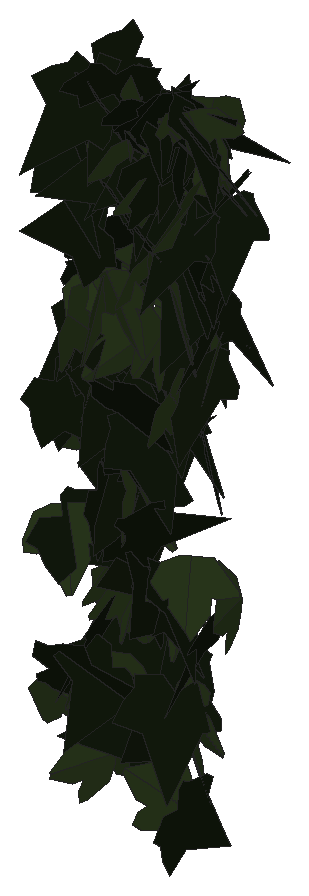
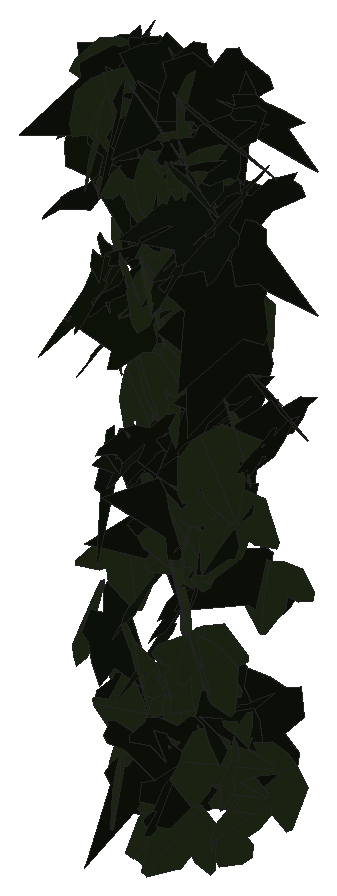
# SketchUp Ruby script. Lengths in inches.
U = 1.inch
M = Sketchup.active_model
def pt(a) = Geom::Point3d.new(a.map { |v| v * U })
def face(e, loops, mat)
  f = e.add_face(loops[0].map { |a| pt(a) })
  loops[1..].each { |l| e.add_face(l.map { |a| pt(a) }).erase! }
  f.material = f.back_material = mat if mat
  f
end
# faces: each face lists its corners as indices into pts; further lists are holes
def faces(e, pts, list, mat = nil) = list.each { |f| face(e, (f[0].is_a?(Array) ? f : [f]).map { |l| l.map { |i| pts[i] } }, mat) }
# xy, xz, yz: faces in a plane at the given z, y or x. An outline is a flat list of corners, or four numbers for a rectangle; further outlines are holes
def ring(l) = l.size == 4 ? [[l[0], l[1]], [l[2], l[1]], [l[2], l[3]], [l[0], l[3]]] : l.each_slice(2).to_a
def flat(e, list, mat, &to3) = list.each { |f| face(e, (f[0].is_a?(Array) ? f : [f]).map { |l| ring(l).map { |u, v| to3.(u, v) } }, mat) }
def xy(e, z, list, mat = nil) = flat(e, list, mat) { |x, y| [x, y, z] }
def xz(e, y, list, mat = nil) = flat(e, list, mat) { |x, z| [x, y, z] }
def yz(e, x, list, mat = nil) = flat(e, list, mat) { |y, z| [x, y, z] }
def lines(e, pts, list) = list.each { |a, b| e.add_line(pt(pts[a]), pt(pts[b])) }
# prism: a flat outline (further loops are holes) pulled along v
def prism(e, loops, v, mat = nil)
  f = face(e, loops, mat); d = Geom::Vector3d.new(v.map { |x| x * U })
  f.pushpull(f.normal.samedirection?(d) ? d.length : -d.length)
end
def box(e, o, s, mat = nil) = prism(e, [[o, [o[0] + s[0], o[1], o[2]], [o[0] + s[0], o[1] + s[1], o[2]], [o[0], o[1] + s[1], o[2]]]], [0, 0, s[2]], mat)
def at(x, y, z, deg = 0) = Geom::Transformation.translation(pt([x, y, z])) * Geom::Transformation.rotation(ORIGIN, Z_AXIS, deg.degrees)
def axes(o, x, y, z) = Geom::Transformation.new([*x, 0, *y, 0, *z, 0, *pt(o).to_a, 1])
def part(name) = M.definitions.add(name)
# library, detail: a bought-in or finely detailed component or shape, given as its bounding box
def library(name, o, s) = part(name).tap { |d| box(d.entities, o, s) }
def detail(e, o, s) = box(e.add_group.entities, o, s)
def put(e, d, t, mat = nil) = e.add_instance(d, t).tap { |i| i.material = mat if mat }
def group(e, t, mat = nil) = e.add_group.tap { |g| g.transformation = t; g.material = mat if mat }.entities
root = M.entities
M.materials.add("efeu1").color = [18, 25, 13]
M.materials.add("efeu2").color = [43, 57, 29]
c1 = part("ivyleaf_9")
p = [[1.54,2.16,1.25],[1.36,2.04,1.19],[-0.21,0.99,0.68],[-0.71,1.11,0.82],[-0.85,0.86,0.67],[-0.8,0.17,0.21],
  [-0.9,-0.01,0.1],[-0.67,-0.16,-0.02],[-0.08,-0.08,-0.05],[-0.03,-0.6,-0.4],[0.65,-0.88,-0.66],[0.83,-0.6,-0.49],
  [1.29,-0.42,-0.43],[1.8125,-0.07,-0.26],[1.21,0.44,0.15]]
faces(c1.entities,p,[[0,1,2,3,4,5,6,7,8,9,10,11,12,13,14]],"efeu1")
c2 = part("ivyleaf_10")
p = [[0,0.5,-0.03],[-0.0625,2.02,-0.43],[-0.19,2.01,-0.46],[-0.54,1.05,-0.29],[-0.52,0.625,-0.18],[-0.83,0.76,-0.28],
  [-1.16,0.64,-0.33],[-1.15,0.33,-0.24],[-0.77,-0.39,0.02],[-0.3,-0.51,0.16],[0.04,-0.48,0.23],[-0.02,2.01,-0.4375],
  [-0.06,2.01,-0.43],[0.04,-0.49,0.23],[0.67,-0.49,0.14],[1.38,0.36,-0.2],[1.375,0.51,-0.24],[0.81,0.65,-0.19],
  [0.62,0.59,-0.15],[0.6,1.09,-0.28],[0.5,1.23,-0.31]]
faces(c2.entities,p,[[0,1,2,3,4,5,6,7,8,9,10],[11,12,0,13,14,15,16,17,18,19,20]],"efeu2")
put(root,c1,axes([35.78,222.67,228.8],[0.26823,-0.25065,-0.33945],[-0.17052,0.30354,-0.35887],[0.38598,0.30828,0.07735]))
put(root,c1,axes([35.7,223.37,232.59],[0.34622,-0.28767,-0.21767],[-0.07063,0.24181,-0.4319],[0.35376,0.32981,0.12681]))
put(root,c1,axes([36.31,222.72,231.47],[-0.08146,-0.0355,-0.49204],[-0.4455,-0.20891,0.08882],[-0.21189,0.45288,0.0024]))
put(root,c2,axes([36.04,223.59,228.91],[-0.1805,-0.4344,0.16947],[-0.02616,-0.172,-0.46875],[0.46555,-0.17809,0.03937]))
put(root,c2,axes([35.7,222.65,224.09],[-0.3103,-0.02254,-0.39142],[0.38813,0.0529,-0.31074],[0.05542,-0.49668,-0.01533]))
put(root,c1,axes([36.125,222.89,229.86],[-0.4834,0.05,-0.11756],[0.11228,-0.05321,-0.48432],[-0.06095,-0.49464,0.04022]))
put(root,c2,axes([36.16,223.65,224.55],[0.13068,0.11386,-0.469],[-0.3279,-0.33557,-0.17284],[-0.35412,0.35274,-0.01304]))
put(root,c2,axes([35.91,223.23,224.48],[-0.00222,0.22987,-0.44402],[0.00293,-0.44401,-0.22988],[-0.49999,-0.00363,0.00063]))
put(root,c1,axes([36.17,222.8,233.44],[-0.4765,-0.15125,0.00835],[-0.00821,-0.00173,-0.49993],[0.15126,-0.47657,-0.00084]))
put(root,c2,axes([35.99,223.16,227.98],[-0.45034,-0.18133,-0.11964],[0.1073,0.05375,-0.48538],[0.18889,-0.46285,-0.0095]))
put(root,c1,axes([35.85,222.97,232.36],[-0.01948,-0.46491,-0.18296],[0.01555,0.18245,-0.46526],[0.49938,-0.02382,0.00735]))
put(root,c1,axes([35.99,223.21,230.57],[0.3227,0.37866,-0.04982],[-0.03386,-0.0366,-0.49751],[-0.38042,0.32447,0.00202]))
put(root,c1,axes([36,223.18,231.07],[0.2778,0.41158,0.05858],[0.03264,0.04864,-0.49656],[-0.41444,0.27971,0.00015]))
put(root,c2,axes([35.93,222.51,226.8],[0.44043,0.21725,0.09393],[0.08386,0.04231,-0.4911],[-0.22133,0.44835,0.00083]))
put(root,c1,axes([36.26,223.58,233.6875],[-0.48953,0.05115,-0.08799],[0.07456,-0.11402,-0.48108],[-0.06928,-0.48413,0.10401]))
put(root,c2,axes([36.12,223.02,229.22],[0.30502,-0.39546,0.02392],[0.01293,-0.02024,-0.49942],[0.39597,0.30529,-0.00212]))
put(root,c1,axes([35.93,222.38,229.02],[0.1908,-0.30196,-0.34988],[-0.0375,0.36716,-0.33732],[0.46064,0.15496,0.11746]))
put(root,c1,axes([36.24,223.14,225.26],[-0.2534,0.19098,-0.38641],[0.2456,-0.30438,-0.3115],[-0.35421,-0.34768,0.06046]))
put(root,c1,axes([35.92,223.39,232.1],[0.4494,-0.21774,0.02514],[0.0212,-0.01391,-0.49936],[0.21816,0.44988,-0.00327]))
put(root,c1,axes([35.84,222.42,224.51],[0.36335,0.00039,0.34348],[0.34324,-0.01919,-0.36307],[0.0129,0.49963,-0.01422]))
put(root,c1,axes([35.94,222.5625,226.84],[0.12166,-0.15399,-0.45988],[0.18407,0.45331,-0.1031],[0.44868,-0.14422,0.16699]))
put(root,c2,axes([36.29,222.87,223.1],[-0.09214,0.0946,0.48225],[0.07301,-0.48257,0.10861],[0.48598,0.09043,0.07511]))
put(root,c2,axes([36.6,223.13,224.27],[0.22876,0.0197,-0.44417],[-0.44327,-0.0286,-0.22956],[-0.03445,0.49879,0.00438]))
put(root,c2,axes([36.28,222.26,230.22],[0.09932,-0.34091,-0.35202],[0.07486,0.36551,-0.33286],[0.48428,0.01342,0.12365]))
put(root,c1,axes([36.3,223.49,233.28],[-0.26529,-0.42283,0.02895],[-0.00108,-0.03348,-0.49888],[0.42381,-0.26476,0.01685]))
put(root,c2,axes([36.35,223.25,225.92],[-0.05732,-0.48356,-0.11349],[0.02307,0.11153,-0.48686],[0.49617,-0.06105,0.00952]))
put(root,c1,axes([36.14,223.05,229.59],[0.09989,-0.29994,-0.38737],[-0.0236,0.39194,-0.30956],[0.48935,0.08012,0.06414]))
put(root,c2,axes([36.06,222.99,230.31],[0.35989,0.15281,0.31165],[0.27231,0.15408,-0.39001],[-0.21524,0.45045,0.02768]))
put(root,c1,axes([35.97,223.09,233.12],[0.21722,-0.2402,0.38094],[0.2648,-0.27398,-0.32375],[0.36427,0.3424,0.00818]))
put(root,c1,axes([36.02,223.16,227.72],[0.32691,-0.2421,0.29071],[0.24717,-0.15419,-0.40636],[0.28641,0.4094,0.01887]))
put(root,c1,axes([36.56,222.85,233.83],[0.14497,0.35763,-0.31794],[-0.0998,-0.3023,-0.38555],[-0.468,0.17525,-0.01627]))
put(root,c1,axes([36.73,223.2,232.3],[-0.36443,-0.11407,0.32277],[-0.29401,-0.13719,-0.38045],[0.17535,-0.46708,0.03291]))
put(root,c2,axes([36.28,223.35,225.76],[-0.38009,-0.11153,-0.30511],[0.29772,0.06829,-0.39585],[0.12997,-0.48259,0.0145]))
put(root,c1,axes([36.42,223.69,224.9375],[-0.28961,-0.36038,-0.1904],[0.13376,0.1366,-0.46201],[0.38502,-0.31853,0.01729]))
put(root,c1,axes([36.45,222.88,224.51],[-0.15382,-0.42719,0.20941],[-0.0591,-0.20122,-0.45389],[0.47207,-0.16438,0.01141]))
put(root,c2,axes([36.55,222.6,230.54],[-0.14671,0.44362,-0.17797],[-0.11799,-0.21402,-0.43621],[-0.4632,-0.086,0.16748]))
put(root,c1,axes([36.46,223.09,228.87],[-0.1355,-0.42773,0.22065],[-0.0327,-0.22052,-0.44755],[0.48018,-0.13572,0.03179]))
put(root,c2,axes([36.55,223.31,225.5625],[-0.30982,-0.37665,-0.1102],[0.07592,0.08023,-0.48765],[0.38503,-0.3189,0.00747]))
put(root,c2,axes([36.46,223.25,232.84],[0.4088,0.28094,0.06285],[0.02139,0.07921,-0.49322],[-0.28709,0.40595,0.05275]))
put(root,c1,axes([36.2,223.49,232.28],[0.42368,-0.22795,0.13612],[0.13552,-0.03477,-0.48003],[0.22832,0.44365,0.03232]))
put(root,c1,axes([36.68,223.45,232.71],[-0.46107,0.02603,-0.19166],[0.17619,-0.14789,-0.44394],[-0.0798,-0.47692,0.1272]))
put(root,c2,axes([36.61,223.51,227],[0.27399,-0.41383,-0.06061],[-0.03218,0.05138,-0.49631],[0.41701,0.27587,0.00152]))
put(root,c1,axes([36.38,223.02,228.65],[-0.07245,-0.15861,-0.46861],[0.15812,0.44134,-0.17383],[0.46877,-0.17338,-0.01379]))
put(root,c2,axes([36.88,222.92,229.81],[-0.25488,-0.20965,0.37561],[-0.26712,-0.26507,-0.32921],[0.33717,-0.36849,0.02312]))
put(root,c2,axes([36.58,223.28,225.9],[0.36585,-0.3298,0.08596],[0.06404,-0.05734,-0.49256],[0.33474,0.37141,0.00029]))
put(root,c2,axes([36.69,222.99,232.72],[-0.09498,-0.48333,-0.08587],[0.00785,0.08596,-0.49249],[0.49083,-0.0949,-0.00874]))
put(root,c1,axes([36.64,222.42,227.53],[0.2242,-0.20144,-0.39894],[-0.31102,0.25018,-0.30112],[0.32094,0.38318,-0.01313]))
put(root,c1,axes([36.93,223.37,223.54],[-0.23005,-0.11338,0.42921],[-0.36503,-0.2268,-0.25557],[0.25264,-0.43094,0.02158]))
put(root,c1,axes([36.6,223.08,227.42],[-0.09735,-0.4093,0.27017],[0.00263,-0.27588,-0.41699],[0.49042,-0.07976,0.05587]))
put(root,c2,axes([36.55,223.32,227.37],[-0.3461,-0.23837,0.27091],[0.22192,0.15539,0.42025],[-0.28454,0.41113,-0.00176]))
put(root,c2,axes([36.625,223.33,233.51],[0.1349,-0.36454,0.3145],[0.2307,-0.23774,-0.37451],[0.42259,0.24615,0.10406]))
put(root,c2,axes([36.64,223.2,227.18],[-0.01911,-0.09533,0.49046],[0.32112,-0.37836,-0.06103],[0.38278,0.31265,0.07569]))
put(root,c1,axes([36.64,222.98,227.66],[0.13764,0.04936,0.47814],[0.35429,0.32571,-0.13561],[-0.32486,0.37614,0.05469]))
put(root,c1,axes([36.61,223.47,231.4375],[0.37818,-0.32426,-0.04289],[-0.03526,0.02477,-0.49814],[0.32517,0.3798,-0.00413]))
put(root,c2,axes([36.98,223.42,230.97],[-0.18558,-0.39095,0.25044],[-0.04019,-0.25516,-0.42811],[0.46254,-0.17902,0.06328]))
put(root,c1,axes([37.23,223.15,232.98],[-0.0778,0.25267,0.42438],[-0.24483,0.35339,-0.25529],[-0.42896,-0.24753,0.06873]))
put(root,c2,axes([36.78,223.08,223.24],[-0.44104,0.01447,-0.23511],[0.23483,-0.012,-0.44126],[-0.01841,-0.49965,0.00379]))
put(root,c2,axes([36.91,223.54,232.71],[-0.05707,-0.39006,0.30757],[0.08537,-0.31269,-0.38071],[0.48934,0.00906,0.10229]))
put(root,c2,axes([36.54,223.34,230.5],[0.07728,0.04512,0.49193],[0.46125,0.17166,-0.08821],[-0.17685,0.46744,-0.01509]))
put(root,c2,axes([36.59,223.1875,227.26],[0.29383,-0.0203,0.40404],[0.40139,0.07697,-0.28803],[-0.05051,0.49362,0.06153]))
put(root,c1,axes([36.93,223.28,226.2],[-0.13324,-0.19137,0.44229],[-0.11916,-0.43156,-0.22262],[0.46695,-0.16473,0.0694]))
put(root,c1,axes([36.86,223.53,223.58],[-0.04076,-0.25659,0.4272],[-0.07856,-0.41996,-0.25974],[0.49211,-0.08829,-0.00608]))
put(root,c1,axes([37.1,223.49,232.71],[-0.39003,-0.26449,0.1671],[-0.10433,-0.1418,-0.46798],[0.29495,-0.39992,0.05542]))
put(root,c1,axes([36.59,222.89,231.76],[0.23828,-0.26841,0.34811],[0.22435,-0.26625,-0.35886],[0.37801,0.32721,-0.00645]))
put(root,c1,axes([36.73,223.27,227.42],[-0.18112,0.08372,0.45846],[0.41994,-0.18398,0.1995],[0.2021,0.45732,-0.00367]))
put(root,c2,axes([37.02,223.54,231.15],[0.22367,-0.447,-0.01284],[-0.00344,0.01263,-0.49983],[0.44717,0.22369,0.00257]))
put(root,c2,axes([36.91,223.34,229.41],[-0.399,0.22899,-0.19586],[0.1296,-0.16299,-0.45457],[-0.27203,-0.41352,0.07071]))
put(root,c2,axes([36.86,222.53,230.79],[-0.39229,0.14922,-0.27175],[0.22152,-0.1717,-0.41406],[-0.21689,-0.44526,0.0686]))
put(root,c1,axes([36.9,223.66,229],[-0.08913,-0.4664,-0.15662],[0.06499,0.14661,-0.47358],[0.48768,-0.10478,0.03449]))
put(root,c1,axes([36.92,222.44,229.2],[0.47066,0.1509,-0.07555],[-0.071,-0.02602,-0.49425],[-0.15309,0.47598,-0.00306]))
put(root,c1,axes([37.09,223.67,224.57],[-0.4346,-0.17992,-0.16957],[0.16172,0.05252,-0.4702],[0.18701,-0.46354,0.01255]))
put(root,c1,axes([36.97,223.18,232.62],[-0.35052,-0.09254,-0.34434],[0.35068,-0.00216,-0.35639],[0.06447,-0.49136,0.06642]))
put(root,c1,axes([37.08,223.6,231.54],[-0.27592,-0.39228,0.14136],[-0.00254,-0.16792,-0.47095],[0.41696,-0.26061,0.09067]))
put(root,c2,axes([37.1,223.53,229.86],[0.48003,-0.13821,-0.02168],[-0.0201,0.00854,-0.49952],[0.13844,0.48044,0.00264]))
put(root,c1,axes([36.97,223.02,228.4],[0.05413,-0.47634,-0.14203],[0.00936,0.14382,-0.47878],[0.49697,0.04918,0.02449]))
put(root,c1,axes([37.11,222.76,233.47],[0.2348,0.36471,0.24871],[0.09341,0.23428,-0.43173],[-0.43144,0.2492,0.04189]))
put(root,c1,axes([37.27,222.73,233.69],[0.18734,0.43004,-0.17313],[-0.08982,-0.14952,-0.46859],[-0.45479,0.20667,0.02123]))
put(root,c2,axes([37.2,222.73,231.16],[0.03596,-0.47879,-0.13953],[0.02642,0.14153,-0.47882],[0.498,0.02706,0.03548]))
put(root,c1,axes([37.03,223.08,225.91],[0.34472,-0.3208,-0.16808],[-0.11321,0.12497,-0.47071],[0.34402,0.36259,0.01352]))
put(root,c2,axes([37.26,223.05,231.44],[-0.20518,0.42461,0.16614],[-0.07599,0.14779,-0.47157],[-0.44958,-0.21877,0.00389]))
put(root,c2,axes([37.11,223.6,225.72],[0.43764,-0.19845,0.13816],[0.12162,-0.06628,-0.48043],[0.209,0.45412,-0.00974]))
put(root,c2,axes([37.21,223.59,229.52],[0.08589,-0.43601,0.22918],[0.12801,-0.20488,-0.43776],[0.47564,0.13387,0.07644]))
put(root,c2,axes([37.41,222.68,230.13],[0.35838,-0.24022,-0.2527],[-0.19289,0.16528,-0.43067],[0.29044,0.40617,0.0258]))
put(root,c2,axes([37.35,223.09,222.7],[-0.01556,0.37087,0.33498],[-0.01236,-0.33533,0.37068],[0.49961,0.00326,0.0196]))
put(root,c2,axes([37.37,222.75,232.49],[-0.10658,-0.48623,-0.04712],[0.00693,0.04671,-0.49776],[0.48846,-0.10675,-0.00321]))
put(root,c1,axes([37.11,222.47,227.05],[0.03145,0.2878,-0.40765],[0.06434,0.40271,0.28928],[0.49484,-0.07066,-0.0117]))
put(root,c1,axes([37.18,222.86,225.97],[0.01805,-0.25323,0.43075],[0.00827,-0.43082,-0.25362],[0.49961,0.01628,-0.01137]))
put(root,c2,axes([37.5,223.15,232.38],[-0.38967,-0.29089,0.11637],[-0.08112,-0.0857,-0.48588],[0.30261,-0.39754,0.0196]))
put(root,c1,axes([37.72,222.3,232.8],[-0.27813,0.32295,0.26143],[-0.1575,0.20917,-0.42596],[-0.3845,-0.3193,-0.01462]))
put(root,c1,axes([37.01,223.54,230.43],[0.3362,-0.3014,0.21477],[0.2429,-0.03921,-0.43527],[0.27923,0.39701,0.12006]))
put(root,c1,axes([37.1875,223.4375,228.68],[0.28646,-0.40341,0.07213],[0.06533,-0.04193,-0.49394],[0.40457,0.29241,0.02869]))
put(root,c1,axes([37.32,222.94,233.16],[0.34279,-0.31809,-0.17695],[-0.098,0.15344,-0.46567],[0.35055,0.35394,0.04285]))
put(root,c2,axes([37.42,223.61,231.33],[0.35231,-0.30766,0.17671],[0.13303,-0.11631,-0.46773],[0.32891,0.37659,-0.0001]))
put(root,c2,axes([37.48,223.1875,232.71],[0.48594,-0.11367,0.03069],[0.0305,-0.00436,-0.49905],[0.11372,0.48689,0.0027]))
put(root,c1,axes([37.56,223.17,233.38],[-0.41535,-0.13779,-0.24187],[0.23482,0.0599,-0.43735],[0.1495,-0.47689,0.01495]))
put(root,c2,axes([37.7,223.51,233.42],[-0.26617,-0.40969,0.10633],[-0.01593,-0.11582,-0.48614],[0.42296,-0.26218,0.0486]))
put(root,c1,axes([37.4,223.54,231.18],[0.15441,-0.45371,0.14248],[0.03156,-0.1397,-0.47905],[0.47451,0.15693,-0.0145]))
put(root,c1,axes([37.57,223.38,230.7],[-0.1429,-0.45163,0.16003],[-0.02116,-0.16088,-0.47294],[0.47868,-0.14194,0.02686]))
put(root,c1,axes([37.73,222.91,233.25],[0.10914,-0.09767,-0.47807],[-0.36427,0.30962,-0.14642],[0.32464,0.38026,-0.00358]))
put(root,c1,axes([37.78,223.3,228.25],[0.24431,-0.03202,-0.43507],[-0.42001,0.11751,-0.2445],[0.11791,0.48494,0.03052]))
put(root,c1,axes([37.47,223.63,230.21],[0.16998,-0.46597,0.06309],[0.02559,-0.05782,-0.49599],[0.46952,0.17185,0.00419]))
put(root,c1,axes([37.48,223.15,231.27],[0.01706,-0.07378,0.49423],[0.23394,-0.4358,-0.07313],[0.44157,0.23374,0.01965]))
put(root,c1,axes([37.54,222.92,226.16],[0.1809,-0.44342,0.1437],[0.04291,-0.13765,-0.47876],[0.46415,0.18555,-0.01175]))
put(root,c1,axes([37.43,223.27,232.93],[0.31502,-0.31709,0.22409],[0.1963,-0.11892,-0.44421],[0.33501,0.36785,0.04956]))
put(root,c2,axes([37.75,222.74,230.75],[-0.29008,0.39323,-0.10595],[0.07135,-0.079,-0.48854],[-0.40096,-0.29855,-0.01028]))
put(root,c2,axes([37.82,222.97,232.2],[-0.10712,0.12571,-0.47193],[-0.06128,-0.48279,-0.1147],[-0.48453,0.03326,0.11884]))
put(root,c1,axes([37.76,222.65,224.63],[-0.27847,-0.36011,-0.20682],[0.1456,0.14853,-0.45468],[0.38891,-0.31346,0.02214]))
put(root,c2,axes([37.93,223.32,233.03],[-0.25629,0.37635,0.20658],[-0.12798,0.16268,-0.45514],[-0.4098,-0.28618,0.01294]))
put(root,c2,axes([38.01,222.82,223.74],[-0.3032,0.30141,0.25928],[-0.19453,0.17192,-0.42732],[-0.34675,-0.36,0.01301]))
put(root,c2,axes([37.89,222.4375,229.45],[0.0044,-0.40281,-0.29618],[0.0454,0.29529,-0.40093],[0.49792,-0.02337,0.03917]))
put(root,c2,axes([37.9,222.93,233.55],[-0.43815,-0.19224,-0.14513],[0.13557,0.05221,-0.47843],[0.19911,-0.4586,0.00638]))
put(root,c1,axes([37.98,222.78,232.09],[-0.44287,-0.13223,-0.19074],[0.22021,-0.1096,-0.43531],[0.07331,-0.46958,0.15531]))
put(root,c1,axes([37.64,223.18,233.33],[0.45481,0.04592,0.20258],[0.1947,0.07571,-0.45427],[-0.07239,0.4921,0.05098]))
put(root,c2,axes([37.92,222.77,226.56],[0.37717,0.32743,-0.02311],[-0.01746,-0.01514,-0.49947],[-0.32778,0.37757,0.00001]))
put(root,c1,axes([38.07,223.08,225.68],[-0.24887,0.26328,-0.34459],[0.22752,-0.25896,-0.36218],[-0.36918,-0.33708,0.00909]))
put(root,c1,axes([38.25,223.01,232.33],[-0.17955,0.46372,0.0522],[-0.0552,0.03443,-0.49575],[-0.46337,-0.18378,0.03883]))
put(root,c2,axes([37.73,222.97,224.4],[-0.15892,0.10687,-0.46187],[0.38076,-0.26144,-0.19151],[-0.28243,-0.41259,0.00171]))
put(root,c1,axes([37.8125,223.12,233.52],[0.14579,-0.45262,0.15452],[0.04753,-0.14703,-0.47552],[0.47591,0.15334,0.00016]))
put(root,c1,axes([38.04,222.85,229.92],[-0.37464,-0.24573,-0.22196],[0.19699,0.10401,-0.44764],[0.26617,-0.42285,0.01888]))
put(root,c1,axes([37.85,222.92,233.4],[0.45384,-0.20726,-0.0327],[-0.02681,0.02001,-0.49888],[0.2081,0.45458,0.00705]))
put(root,c1,axes([37.91,223.39,230.62],[0.37415,-0.29844,-0.14474],[-0.0951,0.11251,-0.47781],[0.31776,0.38507,0.02743]))
put(root,c1,axes([37.97,223.55,232.05],[-0.04086,-0.49767,0.02563],[0.04991,-0.02968,-0.49662],[0.49582,-0.03803,0.05211]))
put(root,c2,axes([37.98,223.65,225.72],[-0.13414,0.06222,0.47763],[0.28392,-0.39031,0.13058],[0.3891,0.30625,0.06939]))
put(root,c1,axes([38.27,222.85,230.53],[-0.36704,0.25748,-0.22132],[0.18348,-0.12381,-0.44834],[-0.28568,-0.41033,-0.0036]))
put(root,c1,axes([38.17,222.26,223.17],[0.06942,-0.09204,-0.48653],[-0.27735,0.39976,-0.1152],[0.41019,0.28587,0.00444]))
put(root,c2,axes([38.12,223.08,230.02],[0.31006,-0.37768,0.10596],[0.06561,-0.08323,-0.48864],[0.38673,0.31691,-0.00205]))
